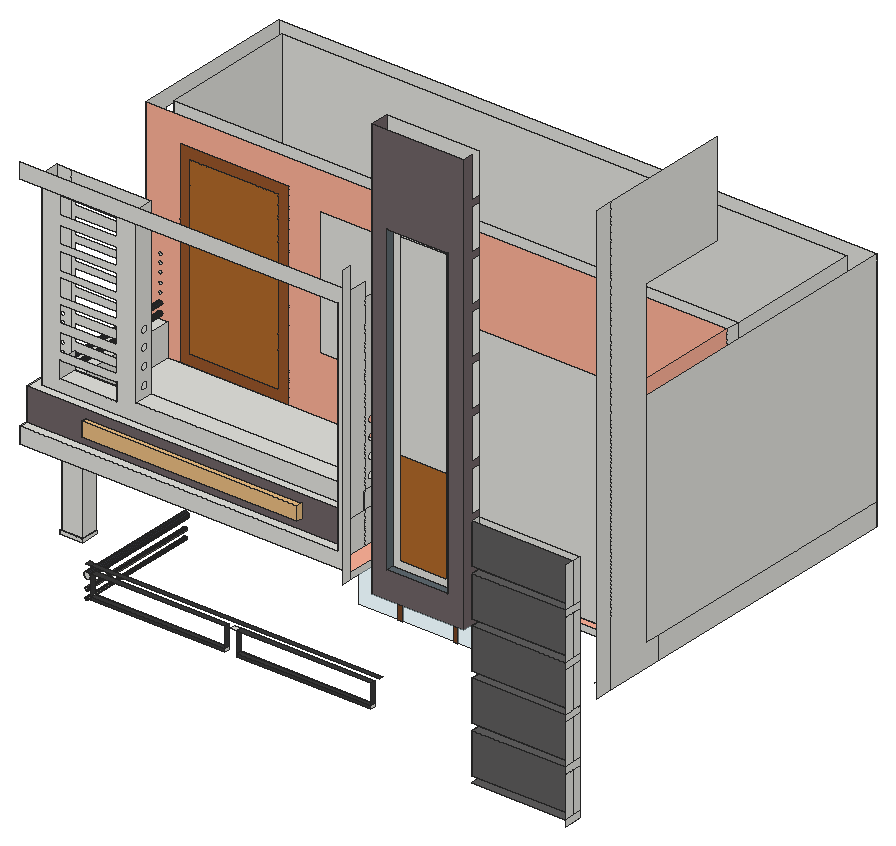
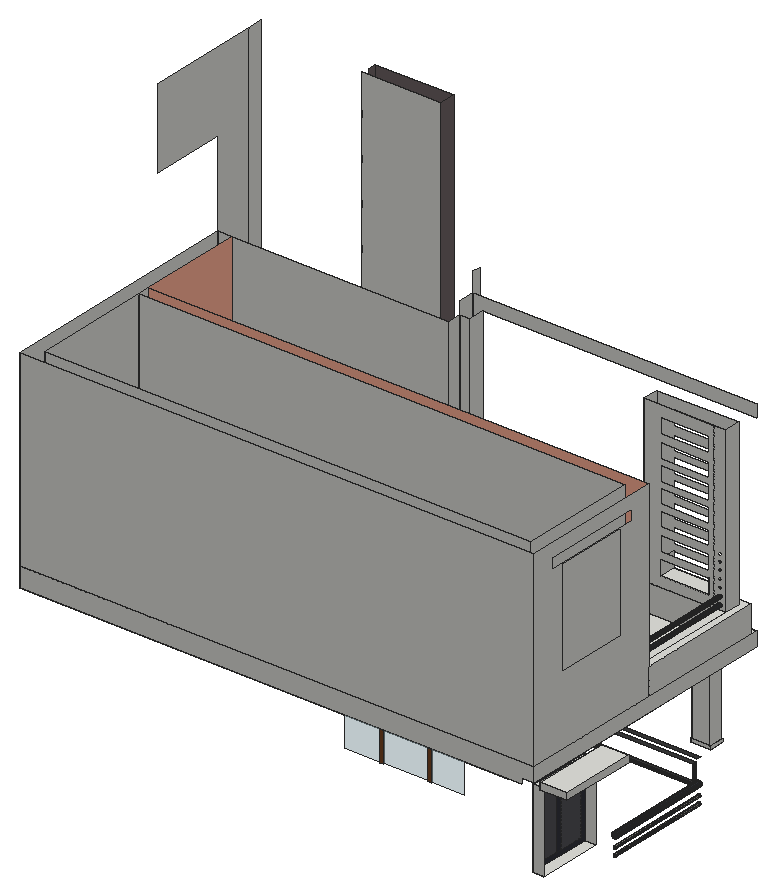
# SketchUp Ruby script. Lengths in inches.
U = 1.inch
M = Sketchup.active_model
def pt(a) = Geom::Point3d.new(a.map { |v| v * U })
def face(e, loops, mat)
  f = e.add_face(loops[0].map { |a| pt(a) })
  loops[1..].each { |l| e.add_face(l.map { |a| pt(a) }).erase! }
  f.material = f.back_material = mat if mat
  f
end
# faces: each face lists its corners as indices into pts; further lists are holes
def faces(e, pts, list, mat = nil) = list.each { |f| face(e, (f[0].is_a?(Array) ? f : [f]).map { |l| l.map { |i| pts[i] } }, mat) }
# xy, xz, yz: faces in a plane at the given z, y or x. An outline is a flat list of corners, or four numbers for a rectangle; further outlines are holes
def ring(l) = l.size == 4 ? [[l[0], l[1]], [l[2], l[1]], [l[2], l[3]], [l[0], l[3]]] : l.each_slice(2).to_a
def flat(e, list, mat, &to3) = list.each { |f| face(e, (f[0].is_a?(Array) ? f : [f]).map { |l| ring(l).map { |u, v| to3.(u, v) } }, mat) }
def xy(e, z, list, mat = nil) = flat(e, list, mat) { |x, y| [x, y, z] }
def xz(e, y, list, mat = nil) = flat(e, list, mat) { |x, z| [x, y, z] }
def yz(e, x, list, mat = nil) = flat(e, list, mat) { |y, z| [x, y, z] }
def lines(e, pts, list) = list.each { |a, b| e.add_line(pt(pts[a]), pt(pts[b])) }
# prism: a flat outline (further loops are holes) pulled along v
def prism(e, loops, v, mat = nil)
  f = face(e, loops, mat); d = Geom::Vector3d.new(v.map { |x| x * U })
  f.pushpull(f.normal.samedirection?(d) ? d.length : -d.length)
end
def box(e, o, s, mat = nil) = prism(e, [[o, [o[0] + s[0], o[1], o[2]], [o[0] + s[0], o[1] + s[1], o[2]], [o[0], o[1] + s[1], o[2]]]], [0, 0, s[2]], mat)
def at(x, y, z, deg = 0) = Geom::Transformation.translation(pt([x, y, z])) * Geom::Transformation.rotation(ORIGIN, Z_AXIS, deg.degrees)
def axes(o, x, y, z) = Geom::Transformation.new([*x, 0, *y, 0, *z, 0, *pt(o).to_a, 1])
def part(name) = M.definitions.add(name)
# library, detail: a bought-in or finely detailed component or shape, given as its bounding box
def library(name, o, s) = part(name).tap { |d| box(d.entities, o, s) }
def detail(e, o, s) = box(e.add_group.entities, o, s)
def put(e, d, t, mat = nil) = e.add_instance(d, t).tap { |i| i.material = mat if mat }
def group(e, t, mat = nil) = e.add_group.tap { |g| g.transformation = t; g.material = mat if mat }.entities
root = M.entities
M.materials.add("[Asphalt New]").color = [112, 100, 103]
M.materials.add("[Blinds Roman Hobbled Blue]").color = [81, 82, 87]
M.materials.add("[Color B02]").color = [255, 178, 153]
M.materials.add("[Color M07]").color = [58, 58, 58]
M.materials.add("[Formica Graystone]").color = [149, 146, 135]
M.materials.add("[Formica Laminate Dark]").color = [50, 53, 60]
M.materials.add("[Formica Speckled Grey]").color = [94, 105, 111]
M.materials.add("[Granite Dark Gray]").color = [96, 95, 95]
M.materials.add("[Granite Dark Gray]1").color = [69, 68, 68]
M.materials.add("[Translucent Glass Safety]").color = [204, 235, 244]
M.materials["[Translucent Glass Safety]"].alpha = 0.5
M.materials.add("[Wood Bamboo]").color = [177, 105, 43]
M.materials.add("[Wood Cherry Original]").color = [152, 86, 42]
M.materials.add("[Wood Veneer 01]").color = [120, 70, 37]
c1 = library("ENGINEER KARAN B",[0.96,0,0],[116.65,7.5625,12])
box(root,[0,159.31,167.09],[16.8125,48.5,4.25])
xy(root,103.37,[[31.31,67.2,103.91,69.74],[110.1,67.2,182.65,69.74]])
xy(root,104.97,[[31.31,67.2,103.91,69.74],[110.1,67.2,182.65,69.74]],"[Color M07]")
xy(root,108.4375,[[261.16,37.37,315.98,42.24]],"[Granite Dark Gray]")
xy(root,111.99,[[261.16,37.37,315.98,42.24]],"[Granite Dark Gray]")
xy(root,116.1,[[107.01,67.2,110.1,69.74]])
xy(root,116.1,[[31.31,67.2,103.91,69.74],[110.1,67.2,182.65,69.74]],"[Color M07]")
xy(root,116.83,[[16.8125,163.89,23.625,204.58]])
xy(root,119.87,[[28.37,67.2,31.31,69.74],[31.31,67.2,187.4,69.74]],"[Color M07]")
xy(root,131.3125,[[16.25,64.74,28.37,65.24],[28.37,64.74,29.06,74.24],[16.25,65.24,16.8125,74.24],[16.8125,65.24,28.37,74.24]])
xy(root,133.125,[[16.25,64.74,16.8125,74.24],[16.8125,64.74,28.37,65.24],[28.37,64.74,29.06,74.24],[16.8125,65.24,28.37,74.24]])
xy(root,133.8125,[[261.16,37.37,315.98,42.24]],"[Granite Dark Gray]")
xy(root,137.37,[[261.16,37.37,315.98,42.24]],"[Granite Dark Gray]")
xy(root,159.1875,[[261.16,37.37,315.98,42.24]],"[Granite Dark Gray]")
xy(root,162.74,[[261.16,37.37,315.98,42.24]],"[Granite Dark Gray]")
xy(root,166.46,[[16.8125,163.89,23.625,204.58]])
xy(root,176.5,[[16.8125,65.24,28.37,74.24],[323.57,74.24,332.57,140.77],[25.8125,140.77,323.57,150.79],[323.57,140.77,332.57,150.79],[25.8125,150.79,323.57,213.09],
  [323.57,150.79,332.57,213.09],[25.8125,213.09,332.57,222.09]])
xy(root,179.875,[[9.125,140.77,16.8125,150.79],[9.125,150.79,16.8125,222.09]])
xy(root,179.875,[[28.37,47.05,28.37,74.24,9.125,74.24,9.125,140.77,323.57,140.77,323.57,74.24,187.4,74.24,187.4,47.05],[9.125,47.05,28.37,65.24],[9.125,65.24,16.8125,74.24]],"[Color B02]")
xy(root,184.5625,[[261.16,37.37,315.98,42.24]],"[Granite Dark Gray]")
xy(root,184.75,[[211.57,32.05,261.16,42.24]],"[Asphalt New]")
xy(root,188.12,[[261.16,37.37,315.98,42.24]],"[Granite Dark Gray]")
xy(root,188.75,[[9.125,47.05,181.15,51.43],[323.83,66.17,323.83,213.34,17.87,213.34,17.87,132.14,9.125,132.14,9.125,222.09,332.57,222.09,332.57,66.17],[20.93,66.17,323.83,132.14],[17.87,132.14,323.83,139.76],[17.87,139.76,323.83,213.34]])
xy(root,199.23,[[219.35,32.05,252.53,36.24]],"[Formica Speckled Grey]")
xy(root,206.0625,[[9.125,51.43,181.15,51.43,181.15,55.96,13.5,55.96,13.5,132.14,9.125,132.14],[13.5,55.96,64.52,66.17],[64.52,55.96,187.4,66.17],[13.5,66.17,20.93,132.14]])
xy(root,209.9375,[[261.16,37.37,315.98,42.24]],"[Granite Dark Gray]")
xy(root,212.53,[[23.59,55.96,54.34,66.17]])
xy(root,213.49,[[261.16,37.37,315.98,42.24]],"[Granite Dark Gray]")
xy(root,215.5625,[[64.52,55.96,181.15,55.96,181.15,57.43,187.4,57.43,187.4,66.17,64.52,66.17],[181.15,55.96,187.4,57.43]])
xz(root,32.05,[[[211.57,184.75,261.16,412.9375],[219.35,199.23,252.53,364.92]]],"[Asphalt New]")
xz(root,36.24,[[[219.35,199.23,252.53,364.92],[223.21,203.1,248.67,361.06]]])
xz(root,36.24,[[223.21,203.1,248.67,254.56]],"[Wood Bamboo]")
xz(root,37.37,[[261.16,111.99,315.98,133.8125],[261.16,137.37,315.98,159.1875],[261.16,162.74,315.98,184.5625],[261.16,188.12,315.98,209.9375],[261.16,213.49,315.98,235.3125]],"[Granite Dark Gray]")
xz(root,42.24,[[261.16,111.99,315.98,133.8125],[261.16,137.37,315.98,159.1875],[261.16,162.74,315.98,184.5625],[211.57,184.75,261.16,412.9375],[261.16,188.12,315.98,209.9375],
  [261.16,213.49,315.98,235.3125]])
xz(root,42.24,[[261.16,108.4375,315.98,111.99],[261.16,133.8125,315.98,137.37],[261.16,159.1875,315.98,162.74],[261.16,184.5625,315.98,188.12],[261.16,209.9375,315.98,213.49]],"[Formica Laminate Dark]")
xz(root,47.05,[[9.125,179.875,187.4,179.875,187.4,316.8125,9.125,316.8125,9.125,308.75,181.15,308.75,181.15,188.75,9.125,188.75]])
xz(root,51.43,[[9.125,188.75,181.15,206.0625]],"[Asphalt New]")
xz(root,55.96,[[[13.5,206.0625,181.15,206.0625,181.15,215.5625,64.52,215.5625,64.52,308.75,13.5,308.75],[23.59,292.4,54.34,301.78],[23.59,212.53,54.34,221.9],[23.59,278.15,54.34,287.53],[23.59,226.03,54.34,235.4],[23.59,265.34,54.34,274.72],[23.59,239.78,54.34,249.15],[23.59,252.65,54.34,262.03]],[181.15,206.0625,187.4,215.5625]])
xz(root,57.43,[[181.15,215.5625,187.4,308.75]])
xz(root,64.74,[[16.25,131.3125,29.06,133.125]])
xz(root,65.24,[[16.8125,133.125,28.37,176.5],[16.8125,176.5,28.37,179.875]])
xz(root,66.17,[[20.93,188.75,187.4,206.0625],[187.4,188.75,323.83,308.75],[323.83,188.75,332.57,308.75],[[13.5,206.0625,20.93,308.75],[16.85,236.5,17.15,236.54,17.42,236.65,17.65,236.83,17.83,237.0625,17.94,237.34,17.98,237.625,17.94,237.92,17.83,238.1875,17.65,238.42,17.42,238.6,17.15,238.71,16.85,238.75,16.5625,238.71,16.29,238.6,16.06,238.42,15.88,238.1875,15.77,237.92,15.73,237.625,15.77,237.34,15.88,237.0625,16.06,236.83,16.29,236.65,16.5625,236.54],[16.85,212.6875,17.15,212.73,17.42,212.84,17.65,213.02,17.83,213.25,17.94,213.52,17.98,213.8125,17.94,214.11,17.83,214.375,17.65,214.61,17.42,214.79,17.15,214.9,16.85,214.9375,16.5625,214.9,16.29,214.79,16.06,214.61,15.88,214.375,15.77,214.11,15.73,213.8125,15.77,213.52,15.88,213.25,16.06,213.02,16.29,212.84,16.5625,212.73],[16.85,232.1875,17.15,232.23,17.42,232.34,17.65,232.52,17.83,232.75,17.94,233.02,17.98,233.3125,17.94,233.61,17.83,233.875,17.65,234.11,17.42,234.29,17.15,234.4,16.85,234.4375,16.5625,234.4,16.29,234.29,16.06,234.11,15.88,233.875,15.77,233.61,15.73,233.3125,15.77,233.02,15.88,232.75,16.06,232.52,16.29,232.34,16.5625,232.23],[16.85,217.6875,17.15,217.73,17.42,217.84,17.65,218.02,17.83,218.25,17.94,218.52,17.98,218.8125,17.94,219.11,17.83,219.375,17.65,219.61,17.42,219.79,17.15,219.9,16.85,219.9375,16.5625,219.9,16.29,219.79,16.06,219.61,15.88,219.375,15.77,219.11,15.73,218.8125,15.77,218.52,15.88,218.25,16.06,218.02,16.29,217.84,16.5625,217.73],[16.85,227.5,17.15,227.54,17.42,227.65,17.65,227.83,17.83,228.0625,17.94,228.34,17.98,228.625,17.94,228.92,17.83,229.1875,17.65,229.42,17.42,229.6,17.15,229.71,16.85,229.75,16.5625,229.71,16.29,229.6,16.06,229.42,15.88,229.1875,15.77,228.92,15.73,228.625,15.77,228.34,15.88,228.0625,16.06,227.83,16.29,227.65,16.5625,227.54],[16.85,222.375,17.15,222.41,17.42,222.53,17.65,222.71,17.83,222.9375,17.94,223.21,17.98,223.5,17.94,223.79,17.83,224.0625,17.65,224.3,17.42,224.48,17.15,224.59,16.85,224.625,16.5625,224.59,16.29,224.48,16.06,224.3,15.88,224.0625,15.77,223.79,15.73,223.5,15.77,223.21,15.88,222.9375,16.06,222.71,16.29,222.53,16.5625,222.41],[16.85,207.75,17.15,207.79,17.42,207.9,17.65,208.08,17.83,208.3125,17.94,208.59,17.98,208.875,17.94,209.17,17.83,209.4375,17.65,209.67,17.42,209.85,17.15,209.96,16.85,210,16.5625,209.96,16.29,209.85,16.06,209.67,15.88,209.4375,15.77,209.17,15.73,208.875,15.77,208.59,15.88,208.3125,16.06,208.08,16.29,207.9,16.5625,207.79]],[[20.93,206.0625,64.52,308.75],[23.59,292.4,54.34,301.78],[23.59,278.15,54.34,287.53],[23.59,265.34,54.34,274.72],[23.59,252.65,54.34,262.03],[23.59,239.78,54.34,249.15],[23.59,226.03,54.34,235.4],[23.59,212.53,54.34,221.9]],
  [64.52,206.0625,187.4,215.5625],[16.85,207.75,17.15,207.79,17.42,207.9,17.65,208.08,17.83,208.3125,17.94,208.59,17.98,208.875,17.94,209.17,17.83,209.4375,17.65,209.67,17.42,209.85,17.15,209.96,16.85,210,16.5625,209.96,16.29,209.85,16.06,209.67,15.88,209.4375,15.77,209.17,15.73,208.875,15.77,208.59,15.88,208.3125,16.06,208.08,16.29,207.9,16.5625,207.79],[16.85,212.6875,17.15,212.73,17.42,212.84,17.65,213.02,17.83,213.25,17.94,213.52,17.98,213.8125,17.94,214.11,17.83,214.375,17.65,214.61,17.42,214.79,17.15,214.9,16.85,214.9375,16.5625,214.9,16.29,214.79,16.06,214.61,15.88,214.375,15.77,214.11,15.73,213.8125,15.77,213.52,15.88,213.25,16.06,213.02,16.29,212.84,16.5625,212.73]])
xz(root,67.2,[[31.31,103.37,103.91,104.97],[110.1,103.37,182.65,104.97]],"[Color M07]")
xz(root,69.74,[[31.31,103.37,103.91,104.97],[110.1,103.37,182.65,104.97]],"[Color M07]")
xz(root,74.24,[[23.42,97.3125,23.65,97.34,23.86,97.43,24.04,97.57,24.18,97.75,24.27,97.96,24.3,98.1875,24.27,98.41,24.18,98.625,24.04,98.81,23.86,98.94,23.65,99.03,23.42,99.0625,23.2,99.03,22.99,98.94,22.81,98.81,22.67,98.625,22.58,98.41,22.55,98.1875,22.58,97.96,22.67,97.75,22.81,97.57,22.99,97.43,23.2,97.34],[23.42,101.875,23.65,101.9,23.86,101.99,24.04,102.13,24.18,102.3125,24.27,102.52,24.3,102.75,24.27,102.98,24.18,103.1875,24.04,103.37,23.86,103.51,23.65,103.59,23.42,103.625,23.2,103.59,22.99,103.51,22.81,103.37,22.67,103.1875,22.58,102.98,22.55,102.75,22.58,102.52,22.67,102.3125,22.81,102.13,22.99,101.99,23.2,101.9],[23.64,107.65,24.1,107.71,24.54,107.89,24.92,108.18,25.2,108.56,25.39,109,25.45,109.46,25.39,109.93,25.2,110.37,24.92,110.75,24.54,111.03,24.1,111.21,23.64,111.28,23.17,111.21,22.73,111.03,22.35,110.75,22.07,110.37,21.88,109.93,21.82,109.46,21.88,109,22.07,108.56,22.35,108.18,22.73,107.89,23.17,107.71],[16.25,131.3125,29.06,133.125],[16.8125,133.125,28.37,176.5],
  [16.8125,176.5,28.37,179.875],[187.4,176.5,323.57,179.875]])
xz(root,132.14,[[9.125,188.75,17.87,206.0625],[17.87,188.75,20.93,206.0625]])
xz(root,132.14,[[[20.93,188.75,27.16,188.75,27.16,294.8125,86.41,294.8125,86.41,188.75,323.83,188.75,323.83,308.75,9.125,308.75,9.125,206.0625,20.93,206.0625],[103.27,219.96,166.59,288.7],[16.85,236.5,16.5625,236.54,16.29,236.65,16.06,236.83,15.88,237.0625,15.77,237.34,15.73,237.625,15.77,237.92,15.88,238.1875,16.06,238.42,16.29,238.6,16.5625,238.71,16.85,238.75,17.15,238.71,17.42,238.6,17.65,238.42,17.83,238.1875,17.94,237.92,17.98,237.625,17.94,237.34,17.83,237.0625,17.65,236.83,17.42,236.65,17.15,236.54],[16.85,232.1875,16.5625,232.23,16.29,232.34,16.06,232.52,15.88,232.75,15.77,233.02,15.73,233.3125,15.77,233.61,15.88,233.875,16.06,234.11,16.29,234.29,16.5625,234.4,16.85,234.4375,17.15,234.4,17.42,234.29,17.65,234.11,17.83,233.875,17.94,233.61,17.98,233.3125,17.94,233.02,17.83,232.75,17.65,232.52,17.42,232.34,17.15,232.23],[16.85,227.5,16.5625,227.54,16.29,227.65,16.06,227.83,15.88,228.0625,15.77,228.34,15.73,228.625,15.77,228.92,15.88,229.1875,16.06,229.42,16.29,229.6,16.5625,229.71,16.85,229.75,17.15,229.71,17.42,229.6,17.65,229.42,17.83,229.1875,17.94,228.92,17.98,228.625,17.94,228.34,17.83,228.0625,17.65,227.83,17.42,227.65,17.15,227.54],[16.85,222.375,16.5625,222.41,16.29,222.53,16.06,222.71,15.88,222.9375,15.77,223.21,15.73,223.5,15.77,223.79,15.88,224.0625,16.06,224.3,16.29,224.48,16.5625,224.59,16.85,224.625,17.15,224.59,17.42,224.48,17.65,224.3,17.83,224.0625,17.94,223.79,17.98,223.5,17.94,223.21,17.83,222.9375,17.65,222.71,17.42,222.53,17.15,222.41],[16.85,217.6875,16.5625,217.73,16.29,217.84,16.06,218.02,15.88,218.25,15.77,218.52,15.73,218.8125,15.77,219.11,15.88,219.375,16.06,219.61,16.29,219.79,16.5625,219.9,16.85,219.9375,17.15,219.9,17.42,219.79,17.65,219.61,17.83,219.375,17.94,219.11,17.98,218.8125,17.94,218.52,17.83,218.25,17.65,218.02,17.42,217.84,17.15,217.73],[16.85,207.75,16.5625,207.79,16.29,207.9,16.06,208.08,15.88,208.3125,15.77,208.59,15.73,208.875,15.77,209.17,15.88,209.4375,16.06,209.67,16.29,209.85,16.5625,209.96,16.85,210,17.15,209.96,17.42,209.85,17.65,209.67,17.83,209.4375,17.94,209.17,17.98,208.875,17.94,208.59,17.83,208.3125,17.65,208.08,17.42,207.9,17.15,207.79],[16.85,212.6875,16.5625,212.73,16.29,212.84,16.06,213.02,15.88,213.25,15.77,213.52,15.73,213.8125,15.77,214.11,15.88,214.375,16.06,214.61,16.29,214.79,16.5625,214.9,16.85,214.9375,17.15,214.9,17.42,214.79,17.65,214.61,17.83,214.375,17.94,214.11,17.98,213.8125,17.94,213.52,17.83,213.25,17.65,213.02,17.42,212.84,17.15,212.73]]],"[Color B02]")
xz(root,132.14,[[33.01,194.6,80.57,288.97]],"[Wood Bamboo]")
xz(root,132.14,[[[27.16,188.75,86.41,294.8125],[33.01,194.6,80.57,288.97]]],"[Wood Cherry Original]")
xz(root,139.76,[[17.87,188.75,323.83,308.75]])
xz(root,140.77,[[16.8125,176.5,323.57,179.875]],"[Color B02]")
xz(root,140.77,[[117.625,98.88,138.77,157.31],[141.24,98.88,168.65,157.31],[171.11,98.88,193.24,157.31]],"[Translucent Glass Safety]")
xz(root,140.77,[[138.77,98.88,141.24,157.31],[168.65,98.88,171.11,157.31]],"[Wood Veneer 01]")
xz(root,163.89,[[16.8125,116.83,23.625,166.46]])
xz(root,204.58,[[16.8125,116.83,23.625,166.46]])
xz(root,213.34,[[17.87,188.75,323.83,308.75]])
xz(root,222.09,[[16.8125,176.5,16.8125,179.875,9.125,179.875,9.125,188.75,332.57,188.75,332.57,176.5],[9.125,188.75,332.57,308.75]])
yz(root,9.125,[[47.05,179.875,222.09,188.75],[51.43,188.75,132.14,206.0625],[[132.14,188.75,222.09,308.75],[153.59,232.83,199.9,293.4],[145.22,293.87,207.97,300.37]]])
yz(root,13.5,[[55.96,206.0625,66.17,308.75]])
yz(root,16.25,[[64.74,131.3125,74.24,133.125]])
yz(root,16.8125,[[65.24,133.125,74.24,176.5],[65.24,176.5,74.24,179.875]])
yz(root,17.87,[[139.76,188.75,213.34,308.75]])
yz(root,20.93,[[66.17,188.75,132.14,206.0625]])
yz(root,23.59,[[55.96,212.53,66.17,221.9]])
yz(root,23.625,[[166.8,119.75,183.12,163.55],[185.99,119.75,201.66,163.55]],"[Blinds Roman Hobbled Blue]")
yz(root,23.625,[[[163.89,116.83,204.58,166.46],[166.8,119.75,201.66,163.55]],[183.12,119.75,185.99,163.55]],"[Formica Laminate Dark]")
yz(root,28.37,[[65.24,133.125,74.24,176.5],[65.24,176.5,74.24,179.875]])
yz(root,29.06,[[64.74,131.3125,74.24,133.125]])
yz(root,31.31,[[67.2,103.37,69.74,104.97]])
yz(root,31.31,[[67.2,104.97,69.74,116.1]],"[Color M07]")
yz(root,54.34,[[55.96,212.53,66.17,221.9]])
yz(root,64.52,[[[55.96,215.5625,66.17,308.75],[61.67,219.21,61.14,219.28,60.64,219.48,60.21,219.8125,59.88,220.24,59.68,220.74,59.61,221.27,59.68,221.8,59.88,222.3,60.21,222.73,60.64,223.06,61.14,223.26,61.67,223.33,62.2,223.26,62.7,223.06,63.13,222.73,63.46,222.3,63.66,221.8,63.73,221.27,63.66,220.74,63.46,220.24,63.13,219.8125,62.7,219.48,62.2,219.28],[61.67,237.71,61.14,237.78,60.64,237.98,60.21,238.3125,59.88,238.74,59.68,239.24,59.61,239.77,59.68,240.3,59.88,240.8,60.21,241.23,60.64,241.56,61.14,241.76,61.67,241.83,62.2,241.76,62.7,241.56,63.13,241.23,63.46,240.8,63.66,240.3,63.73,239.77,63.66,239.24,63.46,238.74,63.13,238.3125,62.7,237.98,62.2,237.78],[61.67,228.64,61.14,228.71,60.64,228.92,60.21,229.25,59.88,229.68,59.68,230.17,59.61,230.71,59.68,231.24,59.88,231.74,60.21,232.17,60.64,232.49,61.14,232.7,61.67,232.77,62.2,232.7,62.7,232.49,63.13,232.17,63.46,231.74,63.66,231.24,63.73,230.71,63.66,230.17,63.46,229.68,63.13,229.25,62.7,228.92,62.2,228.71],[61.67,246.58,61.14,246.65,60.64,246.86,60.21,247.1875,59.88,247.61,59.68,248.11,59.61,248.64,59.68,249.18,59.88,249.68,60.21,250.1,60.64,250.43,61.14,250.64,61.67,250.71,62.2,250.64,62.7,250.43,63.13,250.1,63.46,249.68,63.66,249.18,63.73,248.64,63.66,248.11,63.46,247.61,63.13,247.1875,62.7,246.86,62.2,246.65]]])
yz(root,103.91,[[67.2,103.37,69.74,104.97]])
yz(root,103.91,[[67.2,104.97,69.74,116.1]],"[Color M07]")
yz(root,110.1,[[67.2,103.37,69.74,104.97]])
yz(root,110.1,[[67.2,104.97,69.74,116.1]],"[Color M07]")
yz(root,181.15,[[47.05,188.75,51.43,206.0625],[47.05,206.0625,47.05,308.75,57.43,308.75,57.43,215.5625,55.96,215.5625,55.96,206.0625]])
yz(root,182.65,[[67.2,103.37,69.74,104.97]])
yz(root,182.65,[[67.2,104.97,69.74,116.1]],"[Color M07]")
yz(root,187.4,[[42.24,176.5,47.05,328.8125],[47.05,176.5,74.24,179.875],[47.05,188.75,57.43,206.0625],[57.43,188.75,66.17,206.0625],[47.05,206.0625,55.96,206.0625,55.96,215.5625,57.43,215.5625,57.43,316.8125,47.05,316.8125],
  [55.96,206.0625,57.43,215.5625],[57.43,206.0625,66.17,215.5625],[[57.43,215.5625,66.17,308.75],[61.67,246.58,62.2,246.65,62.7,246.86,63.13,247.1875,63.46,247.61,63.66,248.11,63.73,248.64,63.66,249.18,63.46,249.68,63.13,250.1,62.7,250.43,62.2,250.64,61.67,250.71,61.14,250.64,60.64,250.43,60.21,250.1,59.88,249.68,59.68,249.18,59.61,248.64,59.68,248.11,59.88,247.61,60.21,247.1875,60.64,246.86,61.14,246.65],[61.67,219.21,62.2,219.28,62.7,219.48,63.13,219.8125,63.46,220.24,63.66,220.74,63.73,221.27,63.66,221.8,63.46,222.3,63.13,222.73,62.7,223.06,62.2,223.26,61.67,223.33,61.14,223.26,60.64,223.06,60.21,222.73,59.88,222.3,59.68,221.8,59.61,221.27,59.68,220.74,59.88,220.24,60.21,219.8125,60.64,219.48,61.14,219.28],[61.67,237.71,62.2,237.78,62.7,237.98,63.13,238.3125,63.46,238.74,63.66,239.24,63.73,239.77,63.66,240.3,63.46,240.8,63.13,241.23,62.7,241.56,62.2,241.76,61.67,241.83,61.14,241.76,60.64,241.56,60.21,241.23,59.88,240.8,59.68,240.3,59.61,239.77,59.68,239.24,59.88,238.74,60.21,238.3125,60.64,237.98,61.14,237.78],[61.67,228.64,62.2,228.71,62.7,228.92,63.13,229.25,63.46,229.68,63.66,230.17,63.73,230.71,63.66,231.24,63.46,231.74,63.13,232.17,62.7,232.49,62.2,232.7,61.67,232.77,61.14,232.7,60.64,232.49,60.21,232.17,59.88,231.74,59.68,231.24,59.61,230.71,59.68,230.17,59.88,229.68,60.21,229.25,60.64,228.92,61.14,228.71]]])
yz(root,211.57,[[32.05,184.75,42.24,412.9375]],"[Asphalt New]")
yz(root,219.35,[[32.05,199.23,36.24,364.92]],"[Formica Speckled Grey]")
yz(root,252.53,[[32.05,199.23,36.24,364.92]],"[Formica Speckled Grey]")
yz(root,261.16,[[37.37,188.12,42.24,209.9375],[37.37,213.49,42.24,235.3125]])
yz(root,261.16,[[32.05,184.75,42.24,184.75,42.24,188.12,37.37,188.12,37.37,209.9375,42.24,209.9375,42.24,213.49,37.37,213.49,37.37,235.3125,42.24,235.3125,42.24,238.87,37.37,238.87,37.37,260.6875,42.24,260.6875,42.24,264.24,37.37,264.24,37.37,286.0625,42.24,286.0625,42.24,289.62,37.37,289.62,37.37,311.4375,42.24,311.4375,42.24,314.99,37.37,314.99,37.37,336.8125,42.24,336.8125,42.24,340.37,37.37,340.37,37.37,362.1875,42.24,362.1875,42.24,365.74,37.37,365.74,37.37,387.5625,42.24,387.5625,42.24,391.12,37.37,391.12,37.37,412.9375,32.05,412.9375]],"[Asphalt New]")
yz(root,261.16,[[37.37,111.99,42.24,133.8125],[37.37,137.37,42.24,159.1875],[37.37,162.74,42.24,184.5625]],"[Granite Dark Gray]1")
yz(root,315.98,[[32.62,108.4375,42.24,111.99],[32.62,111.99,37.37,133.8125],[37.37,111.99,42.24,133.8125],[32.62,133.8125,42.24,137.37],[32.62,137.37,37.37,159.1875],
  [37.37,137.37,42.24,159.1875],[32.62,159.1875,42.24,162.74],[32.62,162.74,37.37,184.5625],[37.37,162.74,42.24,184.5625],[32.62,184.5625,42.24,188.12],
  [32.62,188.12,37.37,209.9375],[37.37,188.12,42.24,209.9375],[32.62,209.9375,42.24,213.49],[32.62,213.49,37.37,235.3125],[37.37,213.49,42.24,235.3125]])
yz(root,323.57,[[74.24,176.5,140.77,179.875]],"[Color B02]")
yz(root,323.83,[[132.14,188.75,139.76,308.75],[139.76,188.75,213.34,308.75]])
yz(root,323.83,[[66.17,188.75,132.14,308.75]],"[Color B02]")
yz(root,332.57,[[32.62,176.5,42.24,412.9375],[42.24,176.5,74.24,176.5,74.24,188.75,66.17,188.75,66.17,362.75,114.05,362.75,114.05,412.9375,42.24,412.9375],[74.24,176.5,222.09,188.75],[66.17,188.75,222.09,308.75]])
p = [[23.2,74.24,97.34],[22.99,74.24,97.43],[22.99,140.77,97.43],[23.2,140.77,97.34],[23.42,74.24,97.3125],[23.42,140.77,97.3125],
  [23.65,74.24,97.34],[23.65,140.77,97.34],[23.86,74.24,97.43],[23.86,140.77,97.43],[22.81,74.24,97.57],[22.81,140.77,97.57],
  [24.04,74.24,97.57],[24.04,140.77,97.57],[22.67,74.24,97.75],[22.67,140.77,97.75],[24.18,74.24,97.75],[24.18,140.77,97.75],
  [22.58,74.24,97.96],[22.58,140.77,97.96],[24.27,74.24,97.96],[24.27,140.77,97.96],[22.55,74.24,98.1875],[22.55,140.77,98.1875],
  [24.3,74.24,98.1875],[24.3,140.77,98.1875],[22.58,74.24,98.41],[22.58,140.77,98.41],[24.27,74.24,98.41],[24.27,140.77,98.41],
  [22.67,74.24,98.625],[22.67,140.77,98.625],[24.18,74.24,98.625],[24.18,140.77,98.625],[22.81,74.24,98.81],[22.81,140.77,98.81],
  [24.04,74.24,98.81],[24.04,140.77,98.81],[22.99,74.24,98.94],[22.99,140.77,98.94],[23.86,74.24,98.94],[23.86,140.77,98.94],
  [23.2,74.24,99.03],[23.2,140.77,99.03],[23.65,74.24,99.03],[23.65,140.77,99.03],[23.42,74.24,99.0625],[23.42,140.77,99.0625],
  [23.2,74.24,101.9],[22.99,74.24,101.99],[22.99,140.77,101.99],[23.2,140.77,101.9],[23.42,74.24,101.875],[23.42,140.77,101.875],
  [23.65,74.24,101.9],[23.65,140.77,101.9],[23.86,74.24,101.99],[23.86,140.77,101.99],[22.81,74.24,102.13],[22.81,140.77,102.13],
  [24.04,74.24,102.13],[24.04,140.77,102.13],[22.67,74.24,102.3125],[22.67,140.77,102.3125],[24.18,74.24,102.3125],[24.18,140.77,102.3125],
  [22.58,74.24,102.52],[22.58,140.77,102.52],[24.27,74.24,102.52],[24.27,140.77,102.52],[22.55,74.24,102.75],[22.55,140.77,102.75],
  [24.3,74.24,102.75],[24.3,140.77,102.75],[22.58,74.24,102.98],[22.58,140.77,102.98],[24.27,74.24,102.98],[24.27,140.77,102.98],
  [22.67,74.24,103.1875],[22.67,140.77,103.1875],[24.18,74.24,103.1875],[24.18,140.77,103.1875],[22.81,74.24,103.37],[22.81,140.77,103.37],
  [24.04,74.24,103.37],[24.04,140.77,103.37],[22.99,74.24,103.51],[22.99,140.77,103.51],[23.86,74.24,103.51],[23.86,140.77,103.51],
  [23.2,74.24,103.59],[23.2,140.77,103.59],[23.65,74.24,103.59],[23.65,140.77,103.59],[23.42,74.24,103.625],[23.42,140.77,103.625],
  [23.17,74.24,107.71],[22.73,74.24,107.89],[22.73,140.77,107.89],[23.17,140.77,107.71],[23.64,74.24,107.65],[23.64,140.77,107.65],
  [24.1,74.24,107.71],[24.1,140.77,107.71],[24.54,74.24,107.89],[24.54,140.77,107.89],[22.35,74.24,108.18],[22.35,140.77,108.18],
  [24.92,74.24,108.18],[24.92,140.77,108.18],[22.07,74.24,108.56],[22.07,140.77,108.56],[25.2,74.24,108.56],[25.2,140.77,108.56],
  [21.88,74.24,109],[21.88,140.77,109],[25.39,74.24,109],[25.39,140.77,109],[21.82,74.24,109.46],[21.82,140.77,109.46],
  [25.45,74.24,109.46],[25.45,140.77,109.46],[21.88,74.24,109.93],[21.88,140.77,109.93],[25.39,74.24,109.93],[25.39,140.77,109.93],
  [22.07,74.24,110.37],[22.07,140.77,110.37],[25.2,74.24,110.37],[25.2,140.77,110.37],[22.35,74.24,110.75],[22.35,140.77,110.75],
  [24.92,74.24,110.75],[24.92,140.77,110.75],[22.73,74.24,111.03],[22.73,140.77,111.03],[24.54,74.24,111.03],[24.54,140.77,111.03],
  [23.17,74.24,111.21],[23.17,140.77,111.21],[24.1,74.24,111.21],[24.1,140.77,111.21],[23.64,74.24,111.28],[23.64,140.77,111.28],
  [16.5625,66.17,207.79],[16.29,66.17,207.9],[16.29,132.14,207.9],[16.5625,132.14,207.79],[16.85,66.17,207.75],[16.85,132.14,207.75],
  [17.15,66.17,207.79],[17.15,132.14,207.79],[17.42,66.17,207.9],[17.42,132.14,207.9],[16.06,66.17,208.08],[16.06,132.14,208.08],
  [17.65,66.17,208.08],[17.65,132.14,208.08],[15.88,66.17,208.3125],[15.88,132.14,208.3125],[17.83,66.17,208.3125],[17.83,132.14,208.3125],
  [15.77,66.17,208.59],[15.77,132.14,208.59],[17.94,66.17,208.59],[17.94,132.14,208.59],[15.73,66.17,208.875],[15.73,132.14,208.875],
  [17.98,66.17,208.875],[17.98,132.14,208.875],[15.77,66.17,209.17],[15.77,132.14,209.17],[17.94,66.17,209.17],[17.94,132.14,209.17],
  [15.88,66.17,209.4375],[15.88,132.14,209.4375],[17.83,66.17,209.4375],[17.83,132.14,209.4375],[16.06,66.17,209.67],[16.06,132.14,209.67],
  [17.65,66.17,209.67],[17.65,132.14,209.67],[16.29,66.17,209.85],[16.29,132.14,209.85],[17.42,66.17,209.85],[17.42,132.14,209.85],
  [16.5625,66.17,209.96],[16.5625,132.14,209.96],[17.15,66.17,209.96],[17.15,132.14,209.96],[16.85,66.17,210],[16.85,132.14,210],
  [16.5625,66.17,212.73],[16.29,66.17,212.84],[16.29,132.14,212.84],[16.5625,132.14,212.73],[16.85,66.17,212.6875],[16.85,132.14,212.6875],
  [17.15,66.17,212.73],[17.15,132.14,212.73],[17.42,66.17,212.84],[17.42,132.14,212.84],[16.06,66.17,213.02],[16.06,132.14,213.02],
  [17.65,66.17,213.02],[17.65,132.14,213.02],[15.88,66.17,213.25],[15.88,132.14,213.25],[17.83,66.17,213.25],[17.83,132.14,213.25],
  [15.77,66.17,213.52],[15.77,132.14,213.52],[17.94,66.17,213.52],[17.94,132.14,213.52],[15.73,66.17,213.8125],[15.73,132.14,213.8125],
  [17.98,66.17,213.8125],[17.98,132.14,213.8125],[15.77,66.17,214.11],[15.77,132.14,214.11],[17.94,66.17,214.11],[17.94,132.14,214.11],
  [15.88,66.17,214.375],[15.88,132.14,214.375],[17.83,66.17,214.375],[17.83,132.14,214.375],[16.06,66.17,214.61],[16.06,132.14,214.61],
  [17.65,66.17,214.61],[17.65,132.14,214.61],[16.29,66.17,214.79],[16.29,132.14,214.79],[17.42,66.17,214.79],[17.42,132.14,214.79],
  [16.5625,66.17,214.9],[16.5625,132.14,214.9],[17.15,66.17,214.9],[17.15,132.14,214.9],[16.85,66.17,214.9375],[16.85,132.14,214.9375],
  [25.8125,150.79,176.5],[16.8125,150.79,176.5],[323.57,74.24,176.5],[323.57,42.24,176.5],[187.4,74.24,179.875],[187.4,74.24,188.75]]
faces(root,p,[[0,1,2,3],[4,0,3,5],[6,4,5,7],[8,6,7,9],[1,10,11,2],[12,8,9,13],[10,14,15,11],[16,12,13,17],
  [14,18,19,15],[20,16,17,21],[18,22,23,19],[24,20,21,25],[22,26,27,23],[28,24,25,29],[26,30,31,27],[32,28,29,33],
  [30,34,35,31],[36,32,33,37],[34,38,39,35],[40,36,37,41],[38,42,43,39],[44,40,41,45],[42,46,47,43],[46,44,45,47],
  [48,49,50,51],[52,48,51,53],[54,52,53,55],[56,54,55,57],[49,58,59,50],[60,56,57,61],[58,62,63,59],[64,60,61,65],
  [62,66,67,63],[68,64,65,69],[66,70,71,67],[72,68,69,73],[70,74,75,71],[76,72,73,77],[74,78,79,75],[80,76,77,81],
  [78,82,83,79],[84,80,81,85],[82,86,87,83],[88,84,85,89],[86,90,91,87],[92,88,89,93],[90,94,95,91],[94,92,93,95]],"[Formica Graystone]")
faces(root,p,[[96,97,98,99],[100,96,99,101],[102,100,101,103],[104,102,103,105],[97,106,107,98],[108,104,105,109],[106,110,111,107],[112,108,109,113],
  [110,114,115,111],[116,112,113,117],[114,118,119,115],[120,116,117,121],[118,122,123,119],[124,120,121,125],[122,126,127,123],[128,124,125,129],
  [126,130,131,127],[132,128,129,133],[130,134,135,131],[136,132,133,137],[134,138,139,135],[140,136,137,141],[138,142,143,139],[142,140,141,143],
  [144,145,146,147],[148,144,147,149],[150,148,149,151],[152,150,151,153],[145,154,155,146],[156,152,153,157],[154,158,159,155],[160,156,157,161],
  [158,162,163,159],[164,160,161,165],[162,166,167,163],[168,164,165,169],[166,170,171,167],[172,168,169,173],[170,174,175,171],[176,172,173,177],
  [174,178,179,175],[180,176,177,181],[178,182,183,179],[184,180,181,185],[182,186,187,183],[188,184,185,189],[186,190,191,187],[190,188,189,191],
  [192,193,194,195],[196,192,195,197],[198,196,197,199],[200,198,199,201],[193,202,203,194],[204,200,201,205],[202,206,207,203],[208,204,205,209],
  [206,210,211,207],[212,208,209,213],[210,214,215,211],[216,212,213,217],[214,218,219,215],[220,216,217,221],[218,222,223,219],[224,220,221,225],
  [222,226,227,223],[228,224,225,229],[226,230,231,227],[232,228,229,233],[230,234,235,231],[236,232,233,237],[234,238,239,235],[238,236,237,239]],"[Formica Laminate Dark]")
lines(root,p,[[240,241],[242,243],[244,245]])
put(root,c1,axes([40.25,51.43,194.03],[1,0,0],[0,0,1],[0,-0.24,0]))
